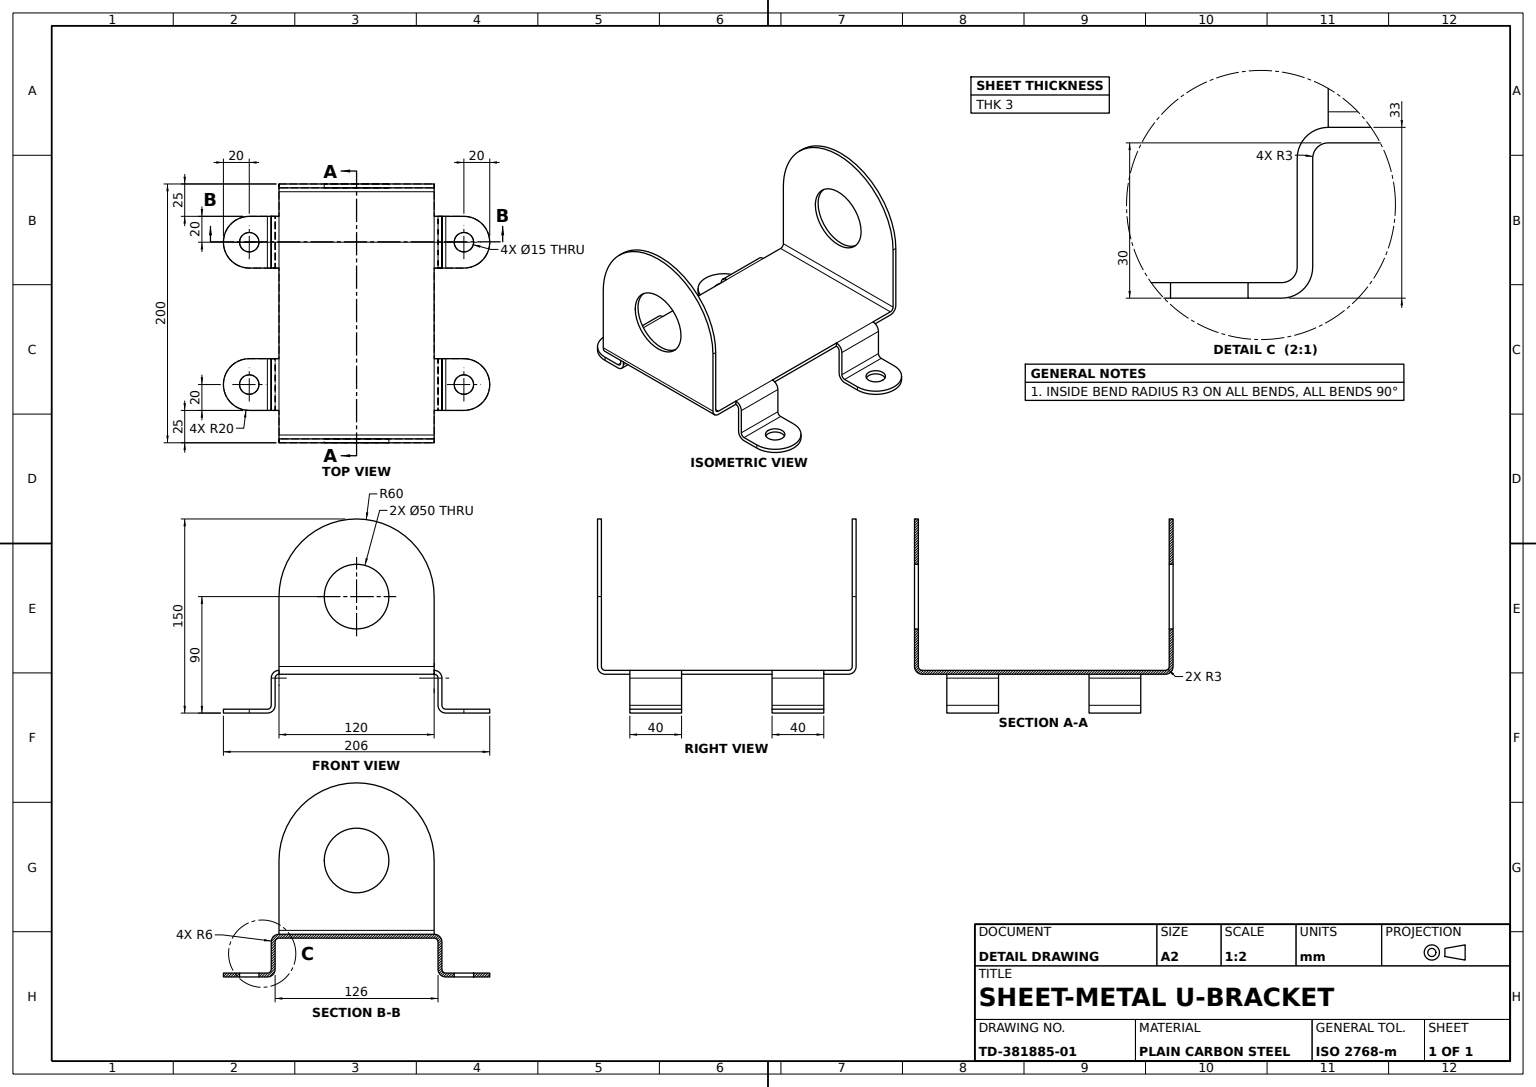
solid
v1 (155,-30,-75.5)
v2 (155,-30,-90.5)
e1 v1 v2 CIRCLE(AX(P(155,-30,-83),D(0,-1,0),D(0,0,-1)),7.5)
e2 v2 v1 CIRCLE(AX(P(155,-30,-83),D(0,-1,0),D(0,0,-1)),7.5)
v3 (135,-30,-83)
v4 (155,-30,-103)
e3 v3 v4 CIRCLE(AX(P(155,-30,-83),D(0,-1,0),D(0,0,1)),20)
v5 (175,-30,-83)
e4 v4 v5 CIRCLE(AX(P(155,-30,-83),D(0,-1,0),D(0,0,1)),20)
v6 (175,-30,-69)
e5 v6 v5 LINE
v7 (135,-30,-69)
e6 v7 v6 LINE
e7 v3 v7 LINE
face PLANE(AX(P(0,-30,0),D(0,1,0),D(0,0,-1))) rev [-e1 -e2] [e3 e4 -e5 -e6 -e7]
v8 (45,-30,-75.5)
v9 (45,-30,-90.5)
e8 v8 v9 CIRCLE(AX(P(45,-30,-83),D(0,1,0),D(0,0,-1)),7.5)
v10 (45,-27,-75.5)
e9 v8 v10 LINE
v11 (45,-27,-90.5)
e10 v10 v11 CIRCLE(AX(P(45,-27,-83),D(0,1,0),D(0,0,-1)),7.5)
e11 v9 v11 LINE
face CYL(AX(P(45,-30,-83),D(0,1,0),D(0,0,1)),7.5) rev [-e8 e9 e10 -e11]
v12 (135,-24,63)
v13 (135,-3,63)
e12 v12 v13 LINE
v14 (175,-3,63)
e13 v14 v13 LINE
v15 (175,-24,63)
e14 v14 v15 LINE
e15 v15 v12 LINE
face PLANE(AX(P(0,0,63),D(0,0,1),D(0,-1,0))) rev [e12 -e13 e14 e15]
v16 (6,0,-60)
v17 (25,0,-60)
e16 v16 v17 LINE
v18 (6,3,-60)
e17 v16 v18 LINE
v19 (25,3,-60)
e18 v18 v19 LINE
e19 v17 v19 LINE
face PLANE(AX(P(3,6,-60),D(0,0,-1),D(-1,0,0))) [-e16 e17 e18 -e19]
v20 (25,-3,-66)
v21 (65,-3,-66)
e20 v20 v21 LINE
v22 (65,-24,-66)
e21 v22 v21 LINE
v23 (25,-24,-66)
e22 v23 v22 LINE
e23 v20 v23 LINE
face PLANE(AX(P(200,0,-66),D(0,0,-1),D(0,-1,0))) [e20 -e21 -e22 -e23]
v24 (197,6,60)
v25 (197,6,-60)
e24 v24 v25 LINE
v26 (194,3,-60)
e25 v26 v25 CIRCLE(AX(P(194,6,-60),D(0,0,1),D(1,0,0)),3)
v27 (194,3,60)
e26 v27 v26 LINE
e27 v27 v24 CIRCLE(AX(P(194,6,60),D(0,0,1),D(1,0,0)),3)
face CYL(AX(P(194,6,60),D(0,0,-1),D(-1,0,0)),3) rev [e24 -e25 -e26 e27]
v28 (0,60,-25)
v29 (0,60,25)
e28 v28 v29 CIRCLE(AX(P(0,60,0),D(1,0,0),D(0,0,-1)),25)
e29 v29 v28 CIRCLE(AX(P(0,60,0),D(1,0,0),D(0,0,-1)),25)
v30 (0,60,60)
v31 (0,6,60)
e30 v30 v31 LINE
v32 (0,120,0)
e31 v30 v32 CIRCLE(AX(P(0,60,0),D(-1,0,0),D(0,0,-1)),60)
v33 (0,60,-60)
e32 v32 v33 CIRCLE(AX(P(0,60,0),D(-1,0,0),D(0,0,-1)),60)
v34 (0,6,-60)
e33 v33 v34 LINE
e34 v31 v34 LINE
face PLANE(AX(P(0,0,60),D(1,0,0),D(0,0,-1))) rev [e28 e29] [-e30 e31 e32 e33 -e34]
v35 (135,-27,-83)
e35 v35 v3 LINE
v36 (155,-27,-103)
e36 v36 v35 CIRCLE(AX(P(155,-27,-83),D(0,1,0),D(0,0,1)),20)
e37 v4 v36 LINE
face CYL(AX(P(155,-30,-83),D(0,1,0),D(0,0,1)),20) [-e35 -e36 -e37 -e3]
v37 (197,60,25)
v38 (197,60,-25)
e38 v37 v38 CIRCLE(AX(P(197,60,0),D(1,0,0),D(0,0,-1)),25)
e39 v38 v37 CIRCLE(AX(P(197,60,0),D(1,0,0),D(0,0,-1)),25)
v39 (197,120,0)
v40 (197,60,-60)
e40 v39 v40 CIRCLE(AX(P(197,60,0),D(-1,0,0),D(0,0,1)),60)
e41 v25 v40 LINE
v41 (197,60,60)
e42 v24 v41 LINE
e43 v41 v39 CIRCLE(AX(P(197,60,0),D(-1,0,0),D(0,0,1)),60)
face PLANE(AX(P(197,0,60),D(-1,0,0),D(0,0,1))) [e38 e39] [e40 -e41 -e24 e42 e43]
v42 (155,-30,90.5)
v43 (155,-27,90.5)
e44 v42 v43 LINE
v44 (155,-30,75.5)
e45 v44 v42 CIRCLE(AX(P(155,-30,83),D(0,1,0),D(0,0,1)),7.5)
v45 (155,-27,75.5)
e46 v44 v45 LINE
e47 v45 v43 CIRCLE(AX(P(155,-27,83),D(0,1,0),D(0,0,1)),7.5)
face CYL(AX(P(155,-30,83),D(0,1,0),D(0,0,1)),7.5) rev [-e44 -e45 e46 e47]
v46 (175,0,-60)
v47 (175,3,-60)
e48 v46 v47 LINE
v48 (175,-3,-63)
e49 v48 v46 CIRCLE(AX(P(175,-3,-60),D(1,0,0),D(0,1,0)),3)
v49 (175,-3,-66)
e50 v48 v49 LINE
e51 v49 v47 CIRCLE(AX(P(175,-3,-60),D(1,0,0),D(0,1,0)),6)
face PLANE(AX(P(175,-3,-60),D(-1,0,0),D(0,-1,0))) rev [-e48 -e49 e50 e51]
v50 (135,3,60)
v51 (175,3,60)
e52 v50 v51 LINE
v52 (135,-3,66)
e53 v52 v50 CIRCLE(AX(P(135,-3,60),D(-1,0,0),D(0,-1,0)),6)
v53 (175,-3,66)
e54 v53 v52 LINE
e55 v51 v53 CIRCLE(AX(P(175,-3,60),D(1,0,0),D(0,-1,0)),6)
face CYL(AX(P(135,-3,60),D(-1,0,0),D(0,0,1)),6) [-e52 -e53 -e54 -e55]
v54 (65,-24,63)
v55 (25,-24,63)
e56 v54 v55 LINE
v56 (65,-30,69)
e57 v56 v54 CIRCLE(AX(P(65,-24,69),D(1,0,0),D(0,0,-1)),6)
v57 (25,-30,69)
e58 v56 v57 LINE
e59 v55 v57 CIRCLE(AX(P(25,-24,69),D(-1,0,0),D(0,0,-1)),6)
face CYL(AX(P(65,-24,69),D(1,0,0),D(0,-1,0)),6) [-e56 -e57 e58 -e59]
v58 (200,60,25)
v59 (200,60,-25)
e60 v58 v59 CIRCLE(AX(P(200,60,0),D(1,0,0),D(0,0,-1)),25)
e61 v59 v58 CIRCLE(AX(P(200,60,0),D(1,0,0),D(0,0,-1)),25)
v60 (200,6,-60)
v61 (200,60,-60)
e62 v60 v61 LINE
v62 (200,120,0)
e63 v61 v62 CIRCLE(AX(P(200,60,0),D(1,0,0),D(0,0,1)),60)
v63 (200,60,60)
e64 v62 v63 CIRCLE(AX(P(200,60,0),D(1,0,0),D(0,0,1)),60)
v64 (200,6,60)
e65 v64 v63 LINE
e66 v64 v60 LINE
face PLANE(AX(P(200,0,60),D(-1,0,0),D(0,0,1))) rev [-e60 -e61] [e62 e63 e64 -e65 e66]
e67 v9 v8 CIRCLE(AX(P(45,-30,-83),D(0,1,0),D(0,0,-1)),7.5)
v65 (45,-30,-103)
v66 (65,-30,-83)
e68 v65 v66 CIRCLE(AX(P(45,-30,-83),D(0,-1,0),D(0,0,1)),20)
v67 (65,-30,-69)
e69 v66 v67 LINE
v68 (25,-30,-69)
e70 v68 v67 LINE
v69 (25,-30,-83)
e71 v68 v69 LINE
e72 v69 v65 CIRCLE(AX(P(45,-30,-83),D(0,-1,0),D(0,0,1)),20)
face PLANE(AX(P(200,-30,0),D(0,1,0),D(0,0,-1))) rev [e8 e67] [e68 e69 -e70 e71 e72]
v70 (6,3,60)
v71 (25,3,60)
e73 v70 v71 LINE
v72 (6,0,60)
e74 v70 v72 LINE
v73 (25,0,60)
e75 v72 v73 LINE
e76 v73 v71 LINE
face PLANE(AX(P(197,6,60),D(0,0,1),D(1,0,0))) [-e73 e74 e75 e76]
v74 (155,-27,-75.5)
e77 v1 v74 LINE
v75 (155,-27,-90.5)
e78 v75 v74 CIRCLE(AX(P(155,-27,-83),D(0,-1,0),D(0,0,-1)),7.5)
e79 v2 v75 LINE
face CYL(AX(P(155,-30,-83),D(0,1,0),D(0,0,1)),7.5) rev [e2 e77 -e78 -e79]
v76 (3,120,0)
v77 (3,60,60)
e80 v76 v77 CIRCLE(AX(P(3,60,0),D(1,0,0),D(0,0,-1)),60)
v78 (3,6,60)
e81 v77 v78 LINE
v79 (3,6,-60)
e82 v78 v79 LINE
v80 (3,60,-60)
e83 v80 v79 LINE
e84 v80 v76 CIRCLE(AX(P(3,60,0),D(1,0,0),D(0,0,-1)),60)
v81 (3,60,25)
v82 (3,60,-25)
e85 v81 v82 CIRCLE(AX(P(3,60,0),D(1,0,0),D(0,0,-1)),25)
e86 v82 v81 CIRCLE(AX(P(3,60,0),D(1,0,0),D(0,0,-1)),25)
face PLANE(AX(P(3,0,60),D(1,0,0),D(0,0,-1))) [e80 e81 e82 -e83 e84] [-e85 -e86]
e87 v40 v61 LINE
e88 v62 v39 LINE
face CYL(AX(P(194,60,0),D(1,0,0),D(0,0,-1)),60) [-e63 -e87 -e40 -e88]
v83 (175,-24,-63)
e89 v48 v83 LINE
v84 (175,-24,-66)
e90 v84 v83 LINE
e91 v49 v84 LINE
face PLANE(AX(P(175,-30,-66),D(-1,0,0),D(0,0,1))) rev [-e50 e89 -e90 -e91]
v85 (25,-3,-63)
e92 v17 v85 CIRCLE(AX(P(25,-3,-60),D(-1,0,0),D(0,1,0)),3)
v86 (65,-3,-63)
e93 v85 v86 LINE
v87 (65,0,-60)
e94 v86 v87 CIRCLE(AX(P(65,-3,-60),D(1,0,0),D(0,1,0)),3)
e95 v87 v17 LINE
face CYL(AX(P(65,-3,-60),D(1,0,0),D(0,0,-1)),3) rev [e92 e93 e94 e95]
v88 (65,-24,-63)
e96 v88 v86 LINE
e97 v22 v88 LINE
e98 v86 v21 LINE
face PLANE(AX(P(65,0,-66),D(1,0,0),D(0,0,-1))) [-e96 -e97 e21 -e98]
v89 (25,-24,-63)
e99 v23 v89 LINE
e100 v85 v89 LINE
e101 v85 v20 LINE
face PLANE(AX(P(25,-30,-66),D(-1,0,0),D(0,0,1))) [e99 -e100 e101 e23]
v90 (135,-24,-63)
e102 v90 v83 LINE
e103 v7 v90 CIRCLE(AX(P(135,-24,-69),D(-1,0,0),D(0,0,1)),6)
e104 v83 v6 CIRCLE(AX(P(175,-24,-69),D(1,0,0),D(0,0,1)),6)
face CYL(AX(P(135,-24,-69),D(-1,0,0),D(0,-1,0)),6) [-e102 -e103 e6 -e104]
v91 (175,-27,-69)
e105 v84 v91 CIRCLE(AX(P(175,-24,-69),D(1,0,0),D(0,0,1)),3)
v92 (135,-27,-69)
e106 v91 v92 LINE
v93 (135,-24,-66)
e107 v92 v93 CIRCLE(AX(P(135,-24,-69),D(-1,0,0),D(0,0,1)),3)
e108 v93 v84 LINE
face CYL(AX(P(135,-24,-69),D(-1,0,0),D(0,-1,0)),3) rev [e105 e106 e107 e108]
v94 (25,-27,-69)
e109 v94 v23 CIRCLE(AX(P(25,-24,-69),D(-1,0,0),D(0,0,1)),3)
e110 v94 v68 LINE
e111 v68 v89 CIRCLE(AX(P(25,-24,-69),D(-1,0,0),D(0,0,1)),6)
face PLANE(AX(P(25,-24,-69),D(1,0,0),D(0,0,-1))) rev [-e109 e110 e111 -e99]
v95 (45,-27,103)
v96 (65,-27,83)
e112 v95 v96 CIRCLE(AX(P(45,-27,83),D(0,1,0),D(0,0,1)),20)
v97 (45,-30,103)
e113 v97 v95 LINE
v98 (65,-30,83)
e114 v98 v97 CIRCLE(AX(P(45,-30,83),D(0,-1,0),D(0,0,1)),20)
e115 v96 v98 LINE
face CYL(AX(P(45,-30,83),D(0,1,0),D(0,0,1)),20) [-e112 -e113 -e114 -e115]
e116 v43 v45 CIRCLE(AX(P(155,-27,83),D(0,1,0),D(0,0,1)),7.5)
v99 (135,-27,83)
v100 (155,-27,103)
e117 v99 v100 CIRCLE(AX(P(155,-27,83),D(0,1,0),D(0,0,1)),20)
v101 (175,-27,83)
e118 v100 v101 CIRCLE(AX(P(155,-27,83),D(0,1,0),D(0,0,1)),20)
v102 (175,-27,69)
e119 v102 v101 LINE
v103 (135,-27,69)
e120 v103 v102 LINE
e121 v99 v103 LINE
face PLANE(AX(P(0,-27,0),D(0,1,0),D(0,0,1))) [-e116 -e47] [e117 e118 -e119 -e120 -e121]
v104 (65,-3,63)
v105 (65,-3,66)
e122 v104 v105 LINE
v106 (65,0,60)
e123 v106 v104 CIRCLE(AX(P(65,-3,60),D(1,0,0),D(0,-1,0)),3)
v107 (65,3,60)
e124 v106 v107 LINE
e125 v107 v105 CIRCLE(AX(P(65,-3,60),D(1,0,0),D(0,-1,0)),6)
face PLANE(AX(P(65,-3,60),D(1,0,0),D(0,1,0))) [-e122 -e123 e124 e125]
v108 (194,0,60)
e126 v108 v64 CIRCLE(AX(P(194,6,60),D(0,0,1),D(-1,0,0)),6)
v109 (194,0,-60)
e127 v108 v109 LINE
e128 v109 v60 CIRCLE(AX(P(194,6,-60),D(0,0,1),D(-1,0,0)),6)
face CYL(AX(P(194,6,60),D(0,0,-1),D(-1,0,0)),6) [-e66 -e126 e127 e128]
v110 (65,-27,69)
e129 v96 v110 LINE
v111 (25,-27,69)
e130 v111 v110 LINE
v112 (25,-27,83)
e131 v111 v112 LINE
e132 v112 v95 CIRCLE(AX(P(45,-27,83),D(0,1,0),D(0,0,1)),20)
v113 (45,-27,90.5)
v114 (45,-27,75.5)
e133 v113 v114 CIRCLE(AX(P(45,-27,83),D(0,-1,0),D(0,0,1)),7.5)
e134 v114 v113 CIRCLE(AX(P(45,-27,83),D(0,-1,0),D(0,0,1)),7.5)
face PLANE(AX(P(200,-27,0),D(0,1,0),D(0,0,1))) [e112 e129 -e130 e131 e132] [e133 e134]
e135 v79 v18 CIRCLE(AX(P(6,6,-60),D(0,0,1),D(1,0,0)),3)
e136 v78 v70 CIRCLE(AX(P(6,6,60),D(0,0,1),D(1,0,0)),3)
e137 v70 v18 LINE
face CYL(AX(P(6,6,60),D(0,0,-1),D(-1,0,0)),3) rev [-e135 -e82 e136 e137]
v115 (175,-24,66)
e138 v53 v115 LINE
v116 (135,-24,66)
e139 v116 v52 LINE
e140 v115 v116 LINE
face PLANE(AX(P(0,0,66),D(0,0,1),D(0,-1,0))) [-e138 e54 -e139 -e140]
e141 v79 v34 LINE
e142 v34 v16 CIRCLE(AX(P(6,6,-60),D(0,0,1),D(-1,0,0)),6)
face PLANE(AX(P(6,0,-60),D(0,0,-1),D(-1,0,0))) [-e141 e135 -e17 -e142]
v117 (25,-3,63)
e143 v117 v73 CIRCLE(AX(P(25,-3,60),D(-1,0,0),D(0,-1,0)),3)
v118 (25,-3,66)
e144 v117 v118 LINE
e145 v118 v71 CIRCLE(AX(P(25,-3,60),D(-1,0,0),D(0,-1,0)),6)
face PLANE(AX(P(25,-3,60),D(1,0,0),D(0,1,0))) rev [-e143 e144 e145 -e76]
e146 v117 v55 LINE
e147 v104 v117 LINE
e148 v54 v104 LINE
face PLANE(AX(P(200,0,63),D(0,0,1),D(0,-1,0))) rev [e56 -e146 -e147 -e148]
v119 (65,-24,66)
e149 v119 v105 LINE
e150 v119 v54 LINE
face PLANE(AX(P(65,0,66),D(-1,0,0),D(0,0,1))) rev [-e149 e150 e148 e122]
e151 v11 v10 CIRCLE(AX(P(45,-27,-83),D(0,1,0),D(0,0,-1)),7.5)
face CYL(AX(P(45,-30,-83),D(0,1,0),D(0,0,1)),7.5) rev [e11 e151 -e9 -e67]
e152 v76 v32 LINE
e153 v33 v80 LINE
face CYL(AX(P(194,60,0),D(-1,0,0),D(0,0,1)),60) [-e152 -e84 -e153 -e32]
v120 (175,-30,69)
v121 (135,-30,69)
e154 v120 v121 LINE
e155 v12 v121 CIRCLE(AX(P(135,-24,69),D(-1,0,0),D(0,0,-1)),6)
e156 v120 v15 CIRCLE(AX(P(175,-24,69),D(1,0,0),D(0,0,-1)),6)
face CYL(AX(P(175,-24,69),D(1,0,0),D(0,-1,0)),6) [e154 -e155 -e15 -e156]
e157 v82 v28 LINE
e158 v81 v29 LINE
face CYL(AX(P(3,60,0),D(-1,0,0),D(0,0,1)),25) rev [e85 e157 -e29 -e158]
e159 v102 v115 CIRCLE(AX(P(175,-24,69),D(1,0,0),D(0,0,-1)),3)
e160 v116 v103 CIRCLE(AX(P(135,-24,69),D(-1,0,0),D(0,0,-1)),3)
face CYL(AX(P(175,-24,69),D(1,0,0),D(0,-1,0)),3) rev [e120 e159 e140 e160]
v122 (65,-27,-83)
e161 v66 v122 LINE
v123 (45,-27,-103)
e162 v65 v123 LINE
e163 v122 v123 CIRCLE(AX(P(45,-27,-83),D(0,1,0),D(0,0,1)),20)
face CYL(AX(P(45,-30,-83),D(0,1,0),D(0,0,1)),20) [-e161 -e68 e162 -e163]
e164 v19 v20 CIRCLE(AX(P(25,-3,-60),D(-1,0,0),D(0,1,0)),6)
v124 (65,3,-60)
e165 v124 v19 LINE
e166 v21 v124 CIRCLE(AX(P(65,-3,-60),D(1,0,0),D(0,1,0)),6)
face CYL(AX(P(65,-3,-60),D(1,0,0),D(0,0,-1)),6) [-e164 -e165 -e166 -e20]
e167 v110 v119 CIRCLE(AX(P(65,-24,69),D(1,0,0),D(0,0,-1)),3)
e168 v110 v56 LINE
face PLANE(AX(P(65,-24,69),D(-1,0,0),D(0,0,1))) rev [-e150 -e167 e168 e57]
e169 v89 v88 LINE
face PLANE(AX(P(200,0,-63),D(0,0,-1),D(0,-1,0))) rev [e169 e96 -e93 e100]
v125 (135,-30,83)
e170 v125 v99 LINE
e171 v103 v121 LINE
e172 v125 v121 LINE
face PLANE(AX(P(135,-30,66),D(1,0,0),D(0,0,-1))) rev [e170 e121 e171 -e172]
v126 (25,-24,66)
e173 v126 v55 LINE
e174 v118 v126 LINE
face PLANE(AX(P(25,-30,66),D(1,0,0),D(0,0,-1))) rev [e146 -e173 -e174 -e144]
v127 (65,-27,-69)
e175 v122 v127 LINE
e176 v127 v67 LINE
face PLANE(AX(P(65,-30,-66),D(-1,0,0),D(0,0,1))) rev [-e69 e161 e175 e176]
e177 v60 v25 LINE
face PLANE(AX(P(194,3,-60),D(0,0,-1),D(-1,0,0))) [e41 e87 -e62 e177]
v128 (175,-30,83)
v129 (155,-30,103)
e178 v128 v129 CIRCLE(AX(P(155,-30,83),D(0,-1,0),D(0,0,1)),20)
e179 v101 v128 LINE
e180 v129 v100 LINE
face CYL(AX(P(155,-30,83),D(0,1,0),D(0,0,1)),20) [-e178 -e179 -e118 -e180]
v130 (25,-27,-83)
e181 v123 v130 CIRCLE(AX(P(45,-27,-83),D(0,1,0),D(0,0,1)),20)
e182 v94 v130 LINE
e183 v127 v94 LINE
face PLANE(AX(P(200,-27,0),D(0,1,0),D(0,0,-1))) [-e151 -e10] [-e175 e163 e181 -e182 -e183]
e184 v37 v58 LINE
e185 v38 v59 LINE
face CYL(AX(P(197,60,0),D(1,0,0),D(0,0,-1)),25) rev [-e184 -e39 e185 e61]
face CYL(AX(P(3,60,0),D(-1,0,0),D(0,0,1)),25) rev [e86 e158 -e28 -e157]
e186 v22 v127 CIRCLE(AX(P(65,-24,-69),D(1,0,0),D(0,0,1)),3)
face CYL(AX(P(25,-24,-69),D(-1,0,0),D(0,-1,0)),3) rev [e186 e183 e109 e22]
e187 v47 v26 LINE
e188 v26 v109 LINE
e189 v46 v109 LINE
face PLANE(AX(P(3,6,-60),D(0,0,-1),D(-1,0,0))) [e48 e187 e188 -e189]
e190 v115 v15 LINE
e191 v14 v53 LINE
face PLANE(AX(P(175,-30,66),D(1,0,0),D(0,0,-1))) [e138 e190 -e14 e191]
e192 v130 v69 LINE
face CYL(AX(P(45,-30,-83),D(0,1,0),D(0,0,1)),20) [-e181 -e162 -e72 -e192]
v131 (135,0,60)
v132 (175,0,60)
e193 v131 v132 LINE
e194 v132 v14 CIRCLE(AX(P(175,-3,60),D(1,0,0),D(0,-1,0)),3)
e195 v13 v131 CIRCLE(AX(P(135,-3,60),D(-1,0,0),D(0,-1,0)),3)
face CYL(AX(P(135,-3,60),D(-1,0,0),D(0,0,1)),3) rev [e193 e194 e13 e195]
e196 v71 v107 LINE
e197 v107 v50 LINE
e198 v51 v27 LINE
v133 (135,3,-60)
e199 v47 v133 LINE
e200 v124 v133 LINE
face PLANE(AX(P(0,3,60),D(0,1,0),D(0,0,1))) [e73 e196 e197 e52 e198 e26 -e187 e199 -e200 e165 -e18 -e137]
v134 (135,-3,-63)
e201 v134 v48 LINE
e202 v90 v134 LINE
face PLANE(AX(P(0,0,-63),D(0,0,-1),D(0,-1,0))) rev [-e201 -e202 e102 -e89]
e203 v111 v57 LINE
v135 (25,-30,83)
e204 v57 v135 LINE
e205 v135 v112 LINE
face PLANE(AX(P(25,-30,103),D(-1,0,0),D(0,0,1))) [e203 e204 e205 -e131]
v136 (135,0,-60)
e206 v46 v136 LINE
e207 v132 v108 LINE
e208 v106 v131 LINE
e209 v73 v106 LINE
e210 v72 v16 LINE
e211 v87 v136 LINE
face PLANE(AX(P(0,0,60),D(0,1,0),D(0,0,1))) rev [-e206 e189 -e127 -e207 -e193 -e208 -e209 -e75 e210 e16 -e95 e211]
v137 (45,-30,90.5)
v138 (45,-30,75.5)
e212 v137 v138 CIRCLE(AX(P(45,-30,83),D(0,-1,0),D(0,0,1)),7.5)
e213 v138 v114 LINE
e214 v137 v113 LINE
face CYL(AX(P(45,-30,83),D(0,1,0),D(0,0,1)),7.5) rev [e212 e213 -e133 -e214]
v139 (135,-3,-66)
e215 v134 v139 LINE
e216 v93 v139 LINE
e217 v93 v90 LINE
face PLANE(AX(P(135,0,-66),D(1,0,0),D(0,0,-1))) rev [e202 e215 -e216 e217]
e218 v139 v49 LINE
e219 v133 v139 CIRCLE(AX(P(135,-3,-60),D(-1,0,0),D(0,1,0)),6)
face CYL(AX(P(175,-3,-60),D(1,0,0),D(0,0,-1)),6) [-e218 -e219 -e199 -e51]
e220 v77 v30 LINE
face CYL(AX(P(0,60,0),D(1,0,0),D(0,0,-1)),60) [-e80 e152 -e31 -e220]
e221 v129 v125 CIRCLE(AX(P(155,-30,83),D(0,-1,0),D(0,0,1)),20)
e222 v120 v128 LINE
e223 v42 v44 CIRCLE(AX(P(155,-30,83),D(0,1,0),D(0,0,1)),7.5)
face PLANE(AX(P(0,-30,0),D(0,1,0),D(0,0,1))) rev [e178 e221 e172 -e154 e222] [e223 e45]
e224 v102 v120 LINE
face PLANE(AX(P(175,-24,69),D(-1,0,0),D(0,0,1))) rev [e156 -e190 -e159 e224]
e225 v31 v78 LINE
e226 v31 v72 CIRCLE(AX(P(6,6,60),D(0,0,1),D(-1,0,0)),6)
face PLANE(AX(P(0,6,60),D(0,0,1),D(1,0,0))) [-e74 -e136 -e225 e226]
face PLANE(AX(P(0,0,-66),D(0,0,-1),D(0,-1,0))) [e218 e91 -e108 e216]
e227 v88 v67 CIRCLE(AX(P(65,-24,-69),D(1,0,0),D(0,0,1)),6)
face CYL(AX(P(25,-24,-69),D(-1,0,0),D(0,-1,0)),6) [-e227 -e169 -e111 e70]
v140 (175,-27,-83)
e228 v5 v140 LINE
e229 v91 v140 LINE
e230 v91 v6 LINE
face PLANE(AX(P(175,-30,-103),D(1,0,0),D(0,0,-1))) [e228 -e229 e230 e5]
e231 v136 v134 CIRCLE(AX(P(135,-3,-60),D(-1,0,0),D(0,1,0)),3)
face CYL(AX(P(175,-3,-60),D(1,0,0),D(0,0,-1)),3) rev [e49 e206 e231 e201]
face CYL(AX(P(197,60,0),D(1,0,0),D(0,0,-1)),25) rev [-e185 -e38 e184 e60]
e232 v131 v50 LINE
face PLANE(AX(P(197,6,60),D(0,0,1),D(1,0,0))) [e208 e232 -e197 -e124]
e233 v105 v118 LINE
face CYL(AX(P(25,-3,60),D(-1,0,0),D(0,0,1)),6) [-e125 -e196 -e145 -e233]
e234 v74 v75 CIRCLE(AX(P(155,-27,-83),D(0,-1,0),D(0,0,-1)),7.5)
face CYL(AX(P(155,-30,-83),D(0,1,0),D(0,0,1)),7.5) rev [-e234 -e77 e1 e79]
e235 v87 v124 LINE
face PLANE(AX(P(65,-3,-60),D(-1,0,0),D(0,-1,0))) rev [e98 e166 -e235 -e94]
face PLANE(AX(P(6,3,60),D(0,0,1),D(1,0,0))) [e30 e225 -e81 e220]
face PLANE(AX(P(194,6,-60),D(0,0,1),D(1,0,0))) rev [e141 -e33 e153 e83]
face PLANE(AX(P(200,6,-60),D(0,0,-1),D(-1,0,0))) [-e188 e25 -e177 -e128]
e236 v63 v41 LINE
e237 v24 v64 LINE
face PLANE(AX(P(194,6,60),D(0,0,1),D(1,0,0))) [e65 e236 -e42 e237]
face CYL(AX(P(25,-3,60),D(-1,0,0),D(0,0,1)),3) rev [e143 e209 e123 e147]
e238 v132 v51 LINE
face PLANE(AX(P(175,-3,60),D(1,0,0),D(0,1,0))) [-e191 -e194 e238 e55]
face CYL(AX(P(6,6,60),D(0,0,-1),D(-1,0,0)),6) [e142 -e210 -e226 e34]
e239 v119 v126 LINE
e240 v126 v111 CIRCLE(AX(P(25,-24,69),D(-1,0,0),D(0,0,-1)),3)
face CYL(AX(P(65,-24,69),D(1,0,0),D(0,-1,0)),3) rev [e167 e239 e240 e130]
face CYL(AX(P(197,60,0),D(1,0,0),D(0,0,-1)),60) [-e236 -e64 e88 -e43]
e241 v108 v27 LINE
face PLANE(AX(P(197,6,60),D(0,0,1),D(1,0,0))) [e241 -e198 -e238 e207]
face PLANE(AX(P(25,-30,-103),D(1,0,0),D(0,0,-1))) rev [e182 e192 -e71 -e110]
face PLANE(AX(P(200,0,66),D(0,0,1),D(0,-1,0))) [e233 e174 -e239 e149]
face PLANE(AX(P(25,-24,69),D(-1,0,0),D(0,0,1))) [-e203 -e240 e173 e59]
e242 v116 v12 LINE
face PLANE(AX(P(135,-24,69),D(-1,0,0),D(0,0,1))) [-e160 e242 e155 -e171]
e243 v13 v52 LINE
face PLANE(AX(P(135,0,66),D(-1,0,0),D(0,0,1))) [-e12 -e242 e139 -e243]
face PLANE(AX(P(65,-24,-69),D(1,0,0),D(0,0,-1))) [e227 -e176 -e186 e97]
e244 v35 v92 LINE
e245 v140 v36 CIRCLE(AX(P(155,-27,-83),D(0,1,0),D(0,0,1)),20)
face PLANE(AX(P(0,-27,0),D(0,1,0),D(0,0,-1))) [e78 e234] [e36 e244 -e106 e229 e245]
e246 v136 v133 LINE
face PLANE(AX(P(135,-3,-60),D(-1,0,0),D(0,-1,0))) [e246 e219 -e215 -e231]
e247 v92 v7 LINE
face PLANE(AX(P(135,-30,-66),D(-1,0,0),D(0,0,1))) [e7 -e247 -e244 e35]
face CYL(AX(P(155,-30,83),D(0,1,0),D(0,0,1)),20) [e180 -e117 -e170 -e221]
e248 v138 v137 CIRCLE(AX(P(45,-30,83),D(0,-1,0),D(0,0,1)),7.5)
face CYL(AX(P(45,-30,83),D(0,1,0),D(0,0,1)),7.5) rev [e214 -e134 -e213 e248]
face CYL(AX(P(155,-30,-83),D(0,1,0),D(0,0,1)),20) [-e228 -e4 e37 -e245]
face CYL(AX(P(155,-30,83),D(0,1,0),D(0,0,1)),7.5) rev [e116 -e46 -e223 e44]
face PLANE(AX(P(135,-24,-69),D(1,0,0),D(0,0,-1))) rev [e247 e103 -e217 -e107]
face PLANE(AX(P(25,-3,-60),D(-1,0,0),D(0,-1,0))) [e164 -e101 -e92 e19]
face PLANE(AX(P(175,-24,-69),D(1,0,0),D(0,0,-1))) [-e105 e90 e104 -e230]
e249 v98 v56 LINE
e250 v97 v135 CIRCLE(AX(P(45,-30,83),D(0,-1,0),D(0,0,1)),20)
face PLANE(AX(P(200,-30,0),D(0,1,0),D(0,0,1))) rev [-e58 -e249 e114 e250 -e204] [-e212 -e248]
face PLANE(AX(P(65,-30,66),D(1,0,0),D(0,0,-1))) [e115 e249 -e168 -e129]
face PLANE(AX(P(175,-30,103),D(-1,0,0),D(0,0,1))) rev [e119 e179 -e222 -e224]
face CYL(AX(P(45,-30,83),D(0,1,0),D(0,0,1)),20) [-e205 -e250 e113 -e132]
face PLANE(AX(P(194,0,60),D(0,0,1),D(1,0,0))) [-e27 -e241 e126 -e237]
face PLANE(AX(P(3,6,-60),D(0,0,-1),D(-1,0,0))) [e200 -e246 -e211 e235]
face PLANE(AX(P(135,-3,60),D(1,0,0),D(0,1,0))) rev [e53 -e232 -e195 e243]
